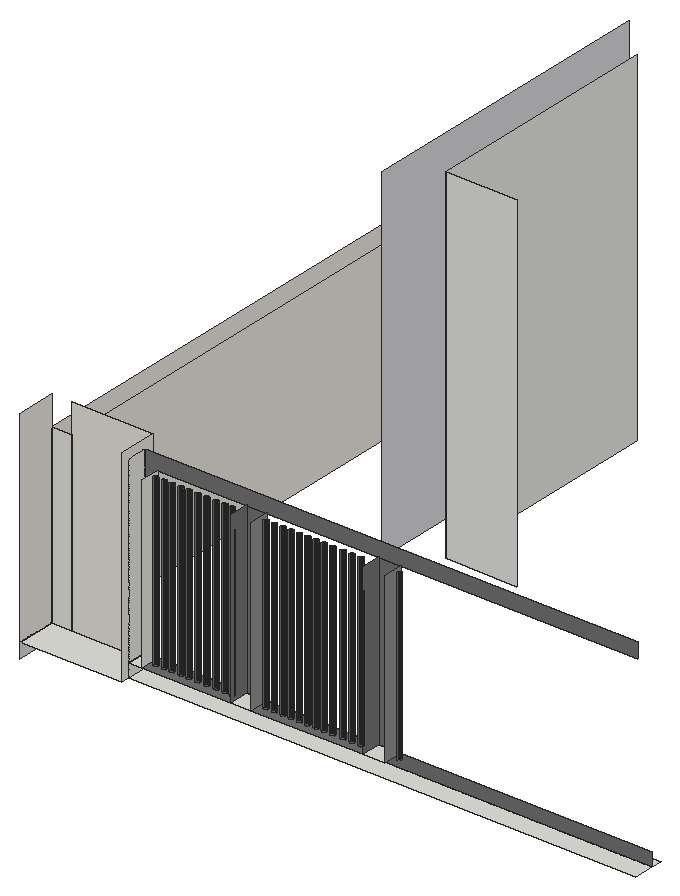
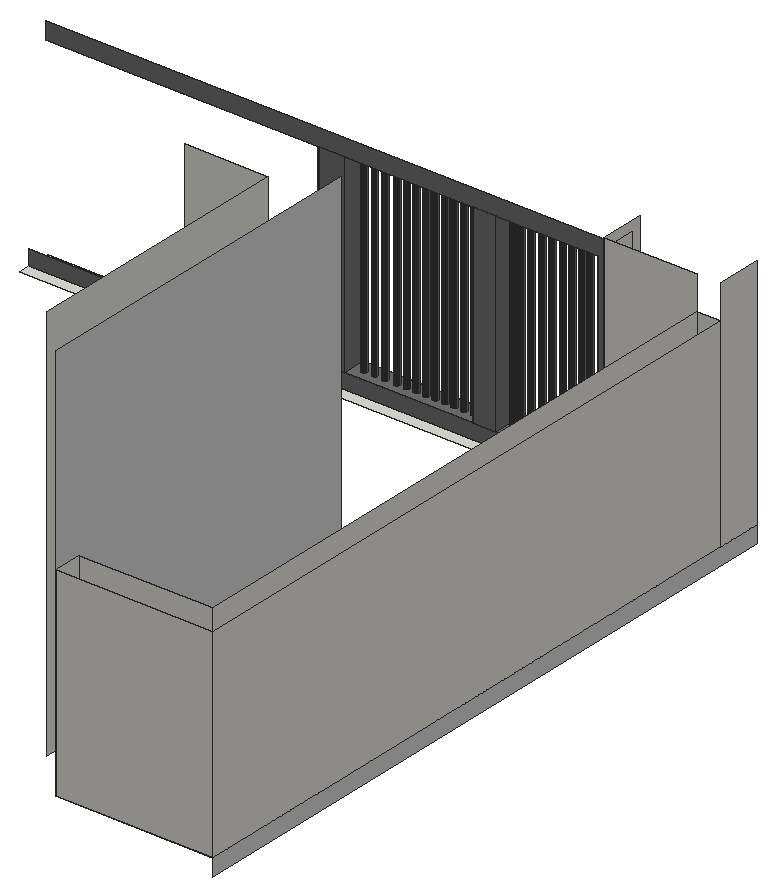
# SketchUp Ruby script. Lengths in inches.
U = 1.inch
M = Sketchup.active_model
def pt(a) = Geom::Point3d.new(a.map { |v| v * U })
def face(e, loops, mat)
  f = e.add_face(loops[0].map { |a| pt(a) })
  loops[1..].each { |l| e.add_face(l.map { |a| pt(a) }).erase! }
  f.material = f.back_material = mat if mat
  f
end
# faces: each face lists its corners as indices into pts; further lists are holes
def faces(e, pts, list, mat = nil) = list.each { |f| face(e, (f[0].is_a?(Array) ? f : [f]).map { |l| l.map { |i| pts[i] } }, mat) }
# xy, xz, yz: faces in a plane at the given z, y or x. An outline is a flat list of corners, or four numbers for a rectangle; further outlines are holes
def ring(l) = l.size == 4 ? [[l[0], l[1]], [l[2], l[1]], [l[2], l[3]], [l[0], l[3]]] : l.each_slice(2).to_a
def flat(e, list, mat, &to3) = list.each { |f| face(e, (f[0].is_a?(Array) ? f : [f]).map { |l| ring(l).map { |u, v| to3.(u, v) } }, mat) }
def xy(e, z, list, mat = nil) = flat(e, list, mat) { |x, y| [x, y, z] }
def xz(e, y, list, mat = nil) = flat(e, list, mat) { |x, z| [x, y, z] }
def yz(e, x, list, mat = nil) = flat(e, list, mat) { |y, z| [x, y, z] }
def lines(e, pts, list) = list.each { |a, b| e.add_line(pt(pts[a]), pt(pts[b])) }
# prism: a flat outline (further loops are holes) pulled along v
def prism(e, loops, v, mat = nil)
  f = face(e, loops, mat); d = Geom::Vector3d.new(v.map { |x| x * U })
  f.pushpull(f.normal.samedirection?(d) ? d.length : -d.length)
end
def box(e, o, s, mat = nil) = prism(e, [[o, [o[0] + s[0], o[1], o[2]], [o[0] + s[0], o[1] + s[1], o[2]], [o[0], o[1] + s[1], o[2]]]], [0, 0, s[2]], mat)
def at(x, y, z, deg = 0) = Geom::Transformation.translation(pt([x, y, z])) * Geom::Transformation.rotation(ORIGIN, Z_AXIS, deg.degrees)
def axes(o, x, y, z) = Geom::Transformation.new([*x, 0, *y, 0, *z, 0, *pt(o).to_a, 1])
def part(name) = M.definitions.add(name)
# library, detail: a bought-in or finely detailed component or shape, given as its bounding box
def library(name, o, s) = part(name).tap { |d| box(d.entities, o, s) }
def detail(e, o, s) = box(e.add_group.entities, o, s)
def put(e, d, t, mat = nil) = e.add_instance(d, t).tap { |i| i.material = mat if mat }
def group(e, t, mat = nil) = e.add_group.tap { |g| g.transformation = t; g.material = mat if mat }.entities
root = M.entities
M.materials.add("[Blinds Vertical Pattern]").color = [212, 212, 214]
M.materials.add("[Color M04]").color = [142, 142, 142]
M.materials.add("[Color M05]").color = [114, 114, 114]
M.materials.add("[Tile Travertine 2 inch]").color = [229, 225, 218]
xy(root,9,[[0,119.71,61.88,143.63],[61.88,125.1875,371.37,137.375],[61.88,137.375,371.37,143.63],[0,143.63,0,479.71,83.3125,479.71,83.3125,464.52,12.5625,464.52,12.5625,143.63]])
xy(root,17.125,[[61.88,125.1875,69.95,137.375],[124.17,125.1875,136.24,137.375],[204.36,125.1875,217.93,137.375]])
xy(root,17.125,[[[69.95,125.1875,124.17,137.375],[119.99,129.51,119.59,129.56,119.21,129.72,118.88,129.97,118.64,130.29,118.48,130.67,118.43,131.07,118.48,131.48,118.64,131.86,118.88,132.18,119.21,132.43,119.59,132.58,119.99,132.64,120.39,132.58,120.77,132.43,121.09,132.18,121.34,131.86,121.5,131.48,121.55,131.07,121.5,130.67,121.34,130.29,121.09,129.97,120.77,129.72,120.39,129.56],[78.3,129.51,77.9,129.56,77.52,129.72,77.2,129.97,76.95,130.29,76.79,130.67,76.74,131.07,76.79,131.48,76.95,131.86,77.2,132.18,77.52,132.43,77.9,132.58,78.3,132.64,78.71,132.58,79.08,132.43,79.41,132.18,79.66,131.86,79.8125,131.48,79.86,131.07,79.8125,130.67,79.66,130.29,79.41,129.97,79.08,129.72,78.71,129.56],[115.49,129.51,115.09,129.56,114.71,129.72,114.38,129.97,114.14,130.29,113.98,130.67,113.93,131.07,113.98,131.48,114.14,131.86,114.38,132.18,114.71,132.43,115.09,132.58,115.49,132.64,115.89,132.58,116.27,132.43,116.59,132.18,116.84,131.86,117,131.48,117.05,131.07,117,130.67,116.84,130.29,116.59,129.97,116.27,129.72,115.89,129.56],[83.3,129.51,82.9,129.56,82.52,129.72,82.2,129.97,81.95,130.29,81.79,130.67,81.74,131.07,81.79,131.48,81.95,131.86,82.2,132.18,82.52,132.43,82.9,132.58,83.3,132.64,83.71,132.58,84.08,132.43,84.41,132.18,84.66,131.86,84.8125,131.48,84.86,131.07,84.8125,130.67,84.66,130.29,84.41,129.97,84.08,129.72,83.71,129.56],[110.11,129.51,109.71,129.56,109.33,129.72,109.01,129.97,108.76,130.29,108.61,130.67,108.55,131.07,108.61,131.48,108.76,131.86,109.01,132.18,109.33,132.43,109.71,132.58,110.11,132.64,110.52,132.58,110.9,132.43,111.22,132.18,111.47,131.86,111.625,131.48,111.68,131.07,111.625,130.67,111.47,130.29,111.22,129.97,110.9,129.72,110.52,129.56],[88.61,129.51,88.21,129.56,87.83,129.72,87.51,129.97,87.26,130.29,87.11,130.67,87.05,131.07,87.11,131.48,87.26,131.86,87.51,132.18,87.83,132.43,88.21,132.58,88.61,132.64,89.02,132.58,89.4,132.43,89.72,132.18,89.97,131.86,90.125,131.48,90.18,131.07,90.125,130.67,89.97,130.29,89.72,129.97,89.4,129.72,89.02,129.56],[104.36,129.51,103.96,129.56,103.58,129.72,103.26,129.97,103.01,130.29,102.86,130.67,102.8,131.07,102.86,131.48,103.01,131.86,103.26,132.18,103.58,132.43,103.96,132.58,104.36,132.64,104.77,132.58,105.15,132.43,105.47,132.18,105.72,131.86,105.875,131.48,105.93,131.07,105.875,130.67,105.72,130.29,105.47,129.97,105.15,129.72,104.77,129.56],[93.43,129.51,93.02,129.56,92.65,129.72,92.32,129.97,92.07,130.29,91.92,130.67,91.86,131.07,91.92,131.48,92.07,131.86,92.32,132.18,92.65,132.43,93.02,132.58,93.43,132.64,93.83,132.58,94.21,132.43,94.53,132.18,94.78,131.86,94.9375,131.48,94.99,131.07,94.9375,130.67,94.78,130.29,94.53,129.97,94.21,129.72,93.83,129.56],[98.93,129.51,98.52,129.56,98.15,129.72,97.82,129.97,97.57,130.29,97.42,130.67,97.36,131.07,97.42,131.48,97.57,131.86,97.82,132.18,98.15,132.43,98.52,132.58,98.93,132.64,99.33,132.58,99.71,132.43,100.03,132.18,100.28,131.86,100.4375,131.48,100.49,131.07,100.4375,130.67,100.28,130.29,100.03,129.97,99.71,129.72,99.33,129.56],[73.24,129.51,72.84,129.56,72.46,129.72,72.13,129.97,71.89,130.29,71.73,130.67,71.68,131.07,71.73,131.48,71.89,131.86,72.13,132.18,72.46,132.43,72.84,132.58,73.24,132.64,73.64,132.58,74.02,132.43,74.34,132.18,74.59,131.86,74.75,131.48,74.8,131.07,74.75,130.67,74.59,130.29,74.34,129.97,74.02,129.72,73.64,129.56]],[[136.24,125.1875,204.36,137.375],[140.68,129.51,140.27,129.56,139.9,129.72,139.57,129.97,139.32,130.29,139.17,130.67,139.11,131.07,139.17,131.48,139.32,131.86,139.57,132.18,139.9,132.43,140.27,132.58,140.68,132.64,141.08,132.58,141.46,132.43,141.78,132.18,142.03,131.86,142.1875,131.48,142.24,131.07,142.1875,130.67,142.03,130.29,141.78,129.97,141.46,129.72,141.08,129.56],[145.74,129.51,145.34,129.56,144.96,129.72,144.63,129.97,144.39,130.29,144.23,130.67,144.18,131.07,144.23,131.48,144.39,131.86,144.63,132.18,144.96,132.43,145.34,132.58,145.74,132.64,146.14,132.58,146.52,132.43,146.84,132.18,147.09,131.86,147.25,131.48,147.3,131.07,147.25,130.67,147.09,130.29,146.84,129.97,146.52,129.72,146.14,129.56],[150.8,129.51,150.4,129.56,150.02,129.72,149.7,129.97,149.45,130.29,149.29,130.67,149.24,131.07,149.29,131.48,149.45,131.86,149.7,132.18,150.02,132.43,150.4,132.58,150.8,132.64,151.21,132.58,151.58,132.43,151.91,132.18,152.16,131.86,152.3125,131.48,152.36,131.07,152.3125,130.67,152.16,130.29,151.91,129.97,151.58,129.72,151.21,129.56],[155.86,129.51,155.46,129.56,155.08,129.72,154.76,129.97,154.51,130.29,154.36,130.67,154.3,131.07,154.36,131.48,154.51,131.86,154.76,132.18,155.08,132.43,155.46,132.58,155.86,132.64,156.27,132.58,156.65,132.43,156.97,132.18,157.22,131.86,157.375,131.48,157.43,131.07,157.375,130.67,157.22,130.29,156.97,129.97,156.65,129.72,156.27,129.56],[160.93,129.51,160.52,129.56,160.15,129.72,159.82,129.97,159.57,130.29,159.42,130.67,159.36,131.07,159.42,131.48,159.57,131.86,159.82,132.18,160.15,132.43,160.52,132.58,160.93,132.64,161.33,132.58,161.71,132.43,162.03,132.18,162.28,131.86,162.4375,131.48,162.49,131.07,162.4375,130.67,162.28,130.29,162.03,129.97,161.71,129.72,161.33,129.56],[165.99,129.51,165.59,129.56,165.21,129.72,164.88,129.97,164.64,130.29,164.48,130.67,164.43,131.07,164.48,131.48,164.64,131.86,164.88,132.18,165.21,132.43,165.59,132.58,165.99,132.64,166.39,132.58,166.77,132.43,167.09,132.18,167.34,131.86,167.5,131.48,167.55,131.07,167.5,130.67,167.34,130.29,167.09,129.97,166.77,129.72,166.39,129.56],[171.05,129.51,170.65,129.56,170.27,129.72,169.95,129.97,169.7,130.29,169.54,130.67,169.49,131.07,169.54,131.48,169.7,131.86,169.95,132.18,170.27,132.43,170.65,132.58,171.05,132.64,171.46,132.58,171.83,132.43,172.16,132.18,172.41,131.86,172.5625,131.48,172.61,131.07,172.5625,130.67,172.41,130.29,172.16,129.97,171.83,129.72,171.46,129.56],[176.11,129.51,175.71,129.56,175.33,129.72,175.01,129.97,174.76,130.29,174.61,130.67,174.55,131.07,174.61,131.48,174.76,131.86,175.01,132.18,175.33,132.43,175.71,132.58,176.11,132.64,176.52,132.58,176.9,132.43,177.22,132.18,177.47,131.86,177.625,131.48,177.68,131.07,177.625,130.67,177.47,130.29,177.22,129.97,176.9,129.72,176.52,129.56],[181.18,129.51,180.77,129.56,180.4,129.72,180.07,129.97,179.82,130.29,179.67,130.67,179.61,131.07,179.67,131.48,179.82,131.86,180.07,132.18,180.4,132.43,180.77,132.58,181.18,132.64,181.58,132.58,181.96,132.43,182.28,132.18,182.53,131.86,182.6875,131.48,182.74,131.07,182.6875,130.67,182.53,130.29,182.28,129.97,181.96,129.72,181.58,129.56],[187.68,129.51,187.27,129.56,186.9,129.72,186.57,129.97,186.32,130.29,186.17,130.67,186.11,131.07,186.17,131.48,186.32,131.86,186.57,132.18,186.9,132.43,187.27,132.58,187.68,132.64,188.08,132.58,188.46,132.43,188.78,132.18,189.03,131.86,189.1875,131.48,189.24,131.07,189.1875,130.67,189.03,130.29,188.78,129.97,188.46,129.72,188.08,129.56],[193.18,129.51,192.77,129.56,192.4,129.72,192.07,129.97,191.82,130.29,191.67,130.67,191.61,131.07,191.67,131.48,191.82,131.86,192.07,132.18,192.4,132.43,192.77,132.58,193.18,132.64,193.58,132.58,193.96,132.43,194.28,132.18,194.53,131.86,194.6875,131.48,194.74,131.07,194.6875,130.67,194.53,130.29,194.28,129.97,193.96,129.72,193.58,129.56],[198.68,129.51,198.27,129.56,197.9,129.72,197.57,129.97,197.32,130.29,197.17,130.67,197.11,131.07,197.17,131.48,197.32,131.86,197.57,132.18,197.9,132.43,198.27,132.58,198.68,132.64,199.08,132.58,199.46,132.43,199.78,132.18,200.03,131.86,200.1875,131.48,200.24,131.07,200.1875,130.67,200.03,130.29,199.78,129.97,199.46,129.72,199.08,129.56]]],"[Color M05]")
xz(root,137.375,[[61.88,9,371.37,17.125],[61.88,17.125,61.88,128.625,362.74,128.625,362.74,119.59,69.95,119.59,69.95,17.125],[124.17,17.125,136.24,119.59],[204.36,17.125,217.93,119.59]],"[Color M05]")
xz(root,143.63,[[0,9,12.5625,116.1875]])
xz(root,143.63,[[12.5625,9,61.88,133.9375]],"[Tile Travertine 2 inch]")
xz(root,309.84,[[107.23,9,151.04,220]])
xz(root,464.52,[[12.5625,9,83.3125,116.1875]],"[Tile Travertine 2 inch]")
xz(root,479.71,[[0,9,83.3125,116.1875]],"[Tile Travertine 2 inch]")
yz(root,0,[[119.71,0,479.71,9]],"[Blinds Vertical Pattern]")
yz(root,0,[[119.71,9,143.63,133.9375],[143.63,9,479.71,116.1875]],"[Tile Travertine 2 inch]")
yz(root,12.5625,[[143.63,9,464.52,116.1875]],"[Tile Travertine 2 inch]")
yz(root,61.88,[[125.1875,9,137.375,17.125],[125.1875,17.125,137.375,128.625]])
yz(root,61.88,[[119.71,9,125.1875,9,125.1875,128.625,137.375,128.625,137.375,9,143.63,9,143.63,133.9375,119.71,133.9375]],"[Tile Travertine 2 inch]")
yz(root,69.95,[[125.1875,17.125,137.375,119.59]])
yz(root,83.3125,[[464.52,9,479.71,116.1875]])
yz(root,83.3125,[[291.34,9,291.34,220,479.71,220,479.71,116.1875,464.52,116.1875,464.52,9]],"[Blinds Vertical Pattern]")
yz(root,107.23,[[309.84,9,455.8,220]])
yz(root,124.17,[[125.1875,17.125,137.375,119.59]],"[Color M05]")
yz(root,136.24,[[125.1875,17.125,137.375,119.59]],"[Color M04]")
yz(root,204.36,[[125.1875,17.125,137.375,119.59]],"[Color M05]")
yz(root,217.93,[[125.1875,17.125,137.375,119.59]],"[Color M04]")
p = [[79.86,131.07,17.125],[79.8125,131.48,17.125],[79.8125,131.48,119.59],[79.86,131.07,119.59],[81.79,131.48,17.125],[81.74,131.07,17.125],
  [81.74,131.07,119.59],[81.79,131.48,119.59],[84.86,131.07,17.125],[84.8125,131.48,17.125],[84.8125,131.48,119.59],[84.86,131.07,119.59],
  [87.11,131.48,17.125],[87.05,131.07,17.125],[87.05,131.07,119.59],[87.11,131.48,119.59],[90.18,131.07,17.125],[90.125,131.48,17.125],
  [90.125,131.48,119.59],[90.18,131.07,119.59],[91.92,131.48,17.125],[91.86,131.07,17.125],[91.86,131.07,119.59],[91.92,131.48,119.59],
  [94.99,131.07,17.125],[94.9375,131.48,17.125],[94.9375,131.48,119.59],[94.99,131.07,119.59],[97.42,131.48,17.125],[97.36,131.07,17.125],
  [97.36,131.07,119.59],[97.42,131.48,119.59],[100.49,131.07,17.125],[100.4375,131.48,17.125],[100.4375,131.48,119.59],[100.49,131.07,119.59],
  [102.86,131.48,17.125],[102.8,131.07,17.125],[102.8,131.07,119.59],[102.86,131.48,119.59],[105.93,131.07,17.125],[105.875,131.48,17.125],
  [105.875,131.48,119.59],[105.93,131.07,119.59],[108.61,131.48,17.125],[108.55,131.07,17.125],[108.55,131.07,119.59],[108.61,131.48,119.59],
  [111.68,131.07,17.125],[111.625,131.48,17.125],[111.625,131.48,119.59],[111.68,131.07,119.59],[113.98,131.48,17.125],[113.93,131.07,17.125],
  [113.93,131.07,119.59],[113.98,131.48,119.59],[117.05,131.07,17.125],[117,131.48,17.125],[117,131.48,119.59],[117.05,131.07,119.59],
  [118.48,131.48,17.125],[118.43,131.07,17.125],[118.43,131.07,119.59],[118.48,131.48,119.59],[121.55,131.07,17.125],[121.5,131.48,17.125],
  [121.5,131.48,119.59],[121.55,131.07,119.59],[139.17,131.48,17.125],[139.11,131.07,17.125],[139.11,131.07,119.59],[139.17,131.48,119.59],
  [142.24,131.07,17.125],[142.1875,131.48,17.125],[142.1875,131.48,119.59],[142.24,131.07,119.59],[144.23,131.48,17.125],[144.18,131.07,17.125],
  [144.18,131.07,119.59],[144.23,131.48,119.59],[147.3,131.07,17.125],[147.25,131.48,17.125],[147.25,131.48,119.59],[147.3,131.07,119.59],
  [149.29,131.48,17.125],[149.24,131.07,17.125],[149.24,131.07,119.59],[149.29,131.48,119.59],[152.36,131.07,17.125],[152.3125,131.48,17.125],
  [152.3125,131.48,119.59],[152.36,131.07,119.59],[154.36,131.48,17.125],[154.3,131.07,17.125],[154.3,131.07,119.59],[154.36,131.48,119.59],
  [157.43,131.07,17.125],[157.375,131.48,17.125],[157.375,131.48,119.59],[157.43,131.07,119.59],[159.42,131.48,17.125],[159.36,131.07,17.125],
  [159.36,131.07,119.59],[159.42,131.48,119.59],[162.49,131.07,17.125],[162.4375,131.48,17.125],[162.4375,131.48,119.59],[162.49,131.07,119.59],
  [164.48,131.48,17.125],[164.43,131.07,17.125],[164.43,131.07,119.59],[164.48,131.48,119.59],[167.55,131.07,17.125],[167.5,131.48,17.125],
  [167.5,131.48,119.59],[167.55,131.07,119.59],[169.54,131.48,17.125],[169.49,131.07,17.125],[169.49,131.07,119.59],[169.54,131.48,119.59],
  [172.61,131.07,17.125],[172.5625,131.48,17.125],[172.5625,131.48,119.59],[172.61,131.07,119.59],[174.61,131.48,17.125],[174.55,131.07,17.125],
  [174.55,131.07,119.59],[174.61,131.48,119.59],[177.68,131.07,17.125],[177.625,131.48,17.125],[177.625,131.48,119.59],[177.68,131.07,119.59],
  [179.67,131.48,17.125],[179.61,131.07,17.125],[179.61,131.07,119.59],[179.67,131.48,119.59],[182.74,131.07,17.125],[182.6875,131.48,17.125],
  [182.6875,131.48,119.59],[182.74,131.07,119.59],[186.17,131.48,17.125],[186.11,131.07,17.125],[186.11,131.07,119.59],[186.17,131.48,119.59],
  [189.24,131.07,17.125],[189.1875,131.48,17.125],[189.1875,131.48,119.59],[189.24,131.07,119.59],[191.67,131.48,17.125],[191.61,131.07,17.125],
  [191.61,131.07,119.59],[191.67,131.48,119.59],[194.74,131.07,17.125],[194.6875,131.48,17.125],[194.6875,131.48,119.59],[194.74,131.07,119.59],
  [197.17,131.48,17.125],[197.11,131.07,17.125],[197.11,131.07,119.59],[197.17,131.48,119.59],[200.24,131.07,17.125],[200.1875,131.48,17.125],
  [200.1875,131.48,119.59],[200.24,131.07,119.59],[220.73,131.48,17.125],[220.68,131.07,17.125],[220.68,131.07,119.59],[220.73,131.48,119.59],
  [71.89,131.86,17.125],[71.73,131.48,17.125],[71.73,131.48,119.59],[71.89,131.86,119.59],[74.75,131.48,17.125],[74.59,131.86,17.125],
  [74.59,131.86,119.59],[74.75,131.48,119.59],[76.95,131.86,17.125],[76.79,131.48,17.125],[76.79,131.48,119.59],[76.95,131.86,119.59],
  [79.66,131.86,17.125],[79.66,131.86,119.59],[81.95,131.86,17.125],[81.95,131.86,119.59],[84.66,131.86,17.125],[84.66,131.86,119.59],
  [87.26,131.86,17.125],[87.26,131.86,119.59],[89.97,131.86,17.125],[89.97,131.86,119.59],[92.07,131.86,17.125],[92.07,131.86,119.59],
  [94.78,131.86,17.125],[94.78,131.86,119.59],[97.57,131.86,17.125],[97.57,131.86,119.59],[100.28,131.86,17.125],[100.28,131.86,119.59],
  [103.01,131.86,17.125],[103.01,131.86,119.59],[105.72,131.86,17.125],[105.72,131.86,119.59],[108.76,131.86,17.125],[108.76,131.86,119.59],
  [111.47,131.86,17.125],[111.47,131.86,119.59],[114.14,131.86,17.125],[114.14,131.86,119.59],[116.84,131.86,17.125],[116.84,131.86,119.59],
  [118.64,131.86,17.125],[118.64,131.86,119.59],[121.34,131.86,17.125],[121.34,131.86,119.59],[139.32,131.86,17.125],[139.32,131.86,119.59],
  [142.03,131.86,17.125],[142.03,131.86,119.59],[144.39,131.86,17.125],[144.39,131.86,119.59],[147.09,131.86,17.125],[147.09,131.86,119.59],
  [149.45,131.86,17.125],[149.45,131.86,119.59],[152.16,131.86,17.125],[152.16,131.86,119.59],[154.51,131.86,17.125],[154.51,131.86,119.59],
  [157.22,131.86,17.125],[157.22,131.86,119.59],[159.57,131.86,17.125],[159.57,131.86,119.59],[162.28,131.86,17.125],[162.28,131.86,119.59],
  [164.64,131.86,17.125],[164.64,131.86,119.59],[167.34,131.86,17.125],[167.34,131.86,119.59],[169.7,131.86,17.125],[169.7,131.86,119.59],
  [172.41,131.86,17.125],[172.41,131.86,119.59],[174.76,131.86,17.125],[174.76,131.86,119.59],[177.47,131.86,17.125],[177.47,131.86,119.59],
  [179.82,131.86,17.125],[179.82,131.86,119.59],[182.53,131.86,17.125],[182.53,131.86,119.59],[186.32,131.86,17.125],[186.32,131.86,119.59],
  [189.03,131.86,17.125],[189.03,131.86,119.59],[191.82,131.86,17.125],[191.82,131.86,119.59],[194.53,131.86,17.125],[194.53,131.86,119.59],
  [197.32,131.86,17.125],[197.32,131.86,119.59],[200.03,131.86,17.125],[200.03,131.86,119.59],[220.89,131.86,17.125],[220.89,131.86,119.59],
  [72.13,132.18,17.125],[72.13,132.18,119.59],[74.34,132.18,17.125],[74.34,132.18,119.59],[77.2,132.18,17.125],[77.2,132.18,119.59],
  [79.41,132.18,17.125],[79.41,132.18,119.59],[82.2,132.18,17.125],[82.2,132.18,119.59],[84.41,132.18,17.125],[84.41,132.18,119.59],
  [87.51,132.18,17.125],[87.51,132.18,119.59],[89.72,132.18,17.125],[89.72,132.18,119.59],[92.32,132.18,17.125],[92.32,132.18,119.59],
  [94.53,132.18,17.125],[94.53,132.18,119.59],[97.82,132.18,17.125],[97.82,132.18,119.59],[100.03,132.18,17.125],[100.03,132.18,119.59],
  [103.26,132.18,17.125],[103.26,132.18,119.59],[105.47,132.18,17.125],[105.47,132.18,119.59],[109.01,132.18,17.125],[109.01,132.18,119.59],
  [111.22,132.18,17.125],[111.22,132.18,119.59],[114.38,132.18,17.125],[114.38,132.18,119.59],[116.59,132.18,17.125],[116.59,132.18,119.59],
  [118.88,132.18,17.125],[118.88,132.18,119.59],[121.09,132.18,17.125],[121.09,132.18,119.59],[139.57,132.18,17.125],[139.57,132.18,119.59],
  [141.78,132.18,17.125],[141.78,132.18,119.59],[144.63,132.18,17.125],[144.63,132.18,119.59],[146.84,132.18,17.125],[146.84,132.18,119.59],
  [149.7,132.18,17.125],[149.7,132.18,119.59],[151.91,132.18,17.125],[151.91,132.18,119.59],[154.76,132.18,17.125],[154.76,132.18,119.59],
  [156.97,132.18,17.125],[156.97,132.18,119.59],[159.82,132.18,17.125],[159.82,132.18,119.59],[162.03,132.18,17.125],[162.03,132.18,119.59],
  [164.88,132.18,17.125],[164.88,132.18,119.59],[167.09,132.18,17.125],[167.09,132.18,119.59],[169.95,132.18,17.125],[169.95,132.18,119.59],
  [172.16,132.18,17.125],[172.16,132.18,119.59],[175.01,132.18,17.125],[175.01,132.18,119.59],[177.22,132.18,17.125],[177.22,132.18,119.59],
  [180.07,132.18,17.125],[180.07,132.18,119.59],[182.28,132.18,17.125],[182.28,132.18,119.59],[186.57,132.18,17.125],[186.57,132.18,119.59],
  [188.78,132.18,17.125],[188.78,132.18,119.59],[192.07,132.18,17.125],[192.07,132.18,119.59],[194.28,132.18,17.125],[194.28,132.18,119.59],
  [197.57,132.18,17.125],[197.57,132.18,119.59],[199.78,132.18,17.125],[199.78,132.18,119.59],[221.13,132.18,17.125],[221.13,132.18,119.59],
  [72.46,132.43,17.125],[72.46,132.43,119.59],[74.02,132.43,17.125],[74.02,132.43,119.59],[77.52,132.43,17.125],[77.52,132.43,119.59],
  [79.08,132.43,17.125],[79.08,132.43,119.59],[82.52,132.43,17.125],[82.52,132.43,119.59],[84.08,132.43,17.125],[84.08,132.43,119.59],
  [87.83,132.43,17.125],[87.83,132.43,119.59],[89.4,132.43,17.125],[89.4,132.43,119.59],[92.65,132.43,17.125],[92.65,132.43,119.59],
  [94.21,132.43,17.125],[94.21,132.43,119.59],[98.15,132.43,17.125],[98.15,132.43,119.59],[99.71,132.43,17.125],[99.71,132.43,119.59],
  [103.58,132.43,17.125],[103.58,132.43,119.59],[105.15,132.43,17.125],[105.15,132.43,119.59],[109.33,132.43,17.125],[109.33,132.43,119.59],
  [110.9,132.43,17.125],[110.9,132.43,119.59],[114.71,132.43,17.125],[114.71,132.43,119.59],[116.27,132.43,17.125],[116.27,132.43,119.59],
  [119.21,132.43,17.125],[119.21,132.43,119.59],[120.77,132.43,17.125],[120.77,132.43,119.59],[139.9,132.43,17.125],[139.9,132.43,119.59],
  [141.46,132.43,17.125],[141.46,132.43,119.59],[144.96,132.43,17.125],[144.96,132.43,119.59],[146.52,132.43,17.125],[146.52,132.43,119.59],
  [150.02,132.43,17.125],[150.02,132.43,119.59],[151.58,132.43,17.125],[151.58,132.43,119.59],[155.08,132.43,17.125],[155.08,132.43,119.59],
  [156.65,132.43,17.125],[156.65,132.43,119.59],[160.15,132.43,17.125],[160.15,132.43,119.59],[161.71,132.43,17.125],[161.71,132.43,119.59],
  [165.21,132.43,17.125],[165.21,132.43,119.59],[166.77,132.43,17.125],[166.77,132.43,119.59],[170.27,132.43,17.125],[170.27,132.43,119.59],
  [171.83,132.43,17.125],[171.83,132.43,119.59],[175.33,132.43,17.125],[175.33,132.43,119.59],[176.9,132.43,17.125],[176.9,132.43,119.59],
  [180.4,132.43,17.125],[180.4,132.43,119.59],[181.96,132.43,17.125],[181.96,132.43,119.59],[186.9,132.43,17.125],[186.9,132.43,119.59],
  [188.46,132.43,17.125],[188.46,132.43,119.59],[192.4,132.43,17.125],[192.4,132.43,119.59],[193.96,132.43,17.125],[193.96,132.43,119.59],
  [197.9,132.43,17.125],[197.9,132.43,119.59],[199.46,132.43,17.125],[199.46,132.43,119.59],[221.46,132.43,17.125],[221.46,132.43,119.59],
  [72.84,132.58,17.125],[72.84,132.58,119.59],[73.64,132.58,17.125],[73.64,132.58,119.59],[77.9,132.58,17.125],[77.9,132.58,119.59],
  [78.71,132.58,17.125],[78.71,132.58,119.59],[82.9,132.58,17.125],[82.9,132.58,119.59],[83.71,132.58,17.125],[83.71,132.58,119.59],
  [88.21,132.58,17.125],[88.21,132.58,119.59],[89.02,132.58,17.125],[89.02,132.58,119.59],[93.02,132.58,17.125],[93.02,132.58,119.59],
  [93.83,132.58,17.125],[93.83,132.58,119.59],[98.52,132.58,17.125],[98.52,132.58,119.59],[99.33,132.58,17.125],[99.33,132.58,119.59],
  [103.96,132.58,17.125],[103.96,132.58,119.59],[104.77,132.58,17.125],[104.77,132.58,119.59],[109.71,132.58,17.125],[109.71,132.58,119.59],
  [110.52,132.58,17.125],[110.52,132.58,119.59],[115.09,132.58,17.125],[115.09,132.58,119.59],[115.89,132.58,17.125],[115.89,132.58,119.59],
  [119.59,132.58,17.125],[119.59,132.58,119.59],[120.39,132.58,17.125],[120.39,132.58,119.59],[140.27,132.58,17.125],[140.27,132.58,119.59],
  [141.08,132.58,17.125],[141.08,132.58,119.59],[145.34,132.58,17.125],[145.34,132.58,119.59],[146.14,132.58,17.125],[146.14,132.58,119.59],
  [150.4,132.58,17.125],[150.4,132.58,119.59],[151.21,132.58,17.125],[151.21,132.58,119.59],[155.46,132.58,17.125],[155.46,132.58,119.59],
  [156.27,132.58,17.125],[156.27,132.58,119.59],[160.52,132.58,17.125],[160.52,132.58,119.59],[161.33,132.58,17.125],[161.33,132.58,119.59],
  [165.59,132.58,17.125],[165.59,132.58,119.59],[166.39,132.58,17.125],[166.39,132.58,119.59],[170.65,132.58,17.125],[170.65,132.58,119.59],
  [171.46,132.58,17.125],[171.46,132.58,119.59],[175.71,132.58,17.125],[175.71,132.58,119.59],[176.52,132.58,17.125],[176.52,132.58,119.59],
  [180.77,132.58,17.125],[180.77,132.58,119.59],[181.58,132.58,17.125],[181.58,132.58,119.59],[187.27,132.58,17.125],[187.27,132.58,119.59],
  [188.08,132.58,17.125],[188.08,132.58,119.59],[192.77,132.58,17.125],[192.77,132.58,119.59],[193.58,132.58,17.125],[193.58,132.58,119.59],
  [198.27,132.58,17.125],[198.27,132.58,119.59],[199.08,132.58,17.125],[199.08,132.58,119.59],[221.84,132.58,17.125],[221.84,132.58,119.59],
  [73.24,132.64,17.125],[73.24,132.64,119.59],[78.3,132.64,17.125],[78.3,132.64,119.59],[83.3,132.64,17.125],[83.3,132.64,119.59],
  [88.61,132.64,17.125],[88.61,132.64,119.59],[93.43,132.64,17.125],[93.43,132.64,119.59],[98.93,132.64,17.125],[98.93,132.64,119.59],
  [104.36,132.64,17.125],[104.36,132.64,119.59],[110.11,132.64,17.125],[110.11,132.64,119.59],[115.49,132.64,17.125],[115.49,132.64,119.59],
  [119.99,132.64,17.125],[119.99,132.64,119.59],[140.68,132.64,17.125],[140.68,132.64,119.59],[145.74,132.64,17.125],[145.74,132.64,119.59],
  [150.8,132.64,17.125],[150.8,132.64,119.59],[155.86,132.64,17.125],[155.86,132.64,119.59],[160.93,132.64,17.125],[160.93,132.64,119.59],
  [165.99,132.64,17.125],[165.99,132.64,119.59],[171.05,132.64,17.125],[171.05,132.64,119.59],[176.11,132.64,17.125],[176.11,132.64,119.59],
  [181.18,132.64,17.125],[181.18,132.64,119.59],[187.68,132.64,17.125],[187.68,132.64,119.59],[193.18,132.64,17.125],[193.18,132.64,119.59],
  [198.68,132.64,17.125],[198.68,132.64,119.59],[222.24,132.64,17.125],[222.24,132.64,119.59]]
faces(root,p,[[0,1,2,3],[4,5,6,7],[8,9,10,11],[12,13,14,15],[16,17,18,19],[20,21,22,23],[24,25,26,27],[28,29,30,31],
  [32,33,34,35],[36,37,38,39],[40,41,42,43],[44,45,46,47],[48,49,50,51],[52,53,54,55],[56,57,58,59],[60,61,62,63],
  [64,65,66,67],[68,69,70,71],[72,73,74,75],[76,77,78,79],[80,81,82,83],[84,85,86,87],[88,89,90,91],[92,93,94,95],
  [96,97,98,99],[100,101,102,103],[104,105,106,107],[108,109,110,111],[112,113,114,115],[116,117,118,119],[120,121,122,123],[124,125,126,127],
  [128,129,130,131],[132,133,134,135],[136,137,138,139],[140,141,142,143],[144,145,146,147],[148,149,150,151],[152,153,154,155],[156,157,158,159],
  [160,161,162,163],[164,165,166,167],[168,169,170,171],[172,173,174,175],[176,177,178,179],[1,180,181,2],[182,4,7,183],[9,184,185,10],
  [186,12,15,187],[17,188,189,18],[190,20,23,191],[25,192,193,26],[194,28,31,195],[33,196,197,34],[198,36,39,199],[41,200,201,42],
  [202,44,47,203],[49,204,205,50],[206,52,55,207],[57,208,209,58],[210,60,63,211],[65,212,213,66],[214,68,71,215],[73,216,217,74],
  [218,76,79,219],[81,220,221,82],[222,84,87,223],[89,224,225,90],[226,92,95,227],[97,228,229,98],[230,100,103,231],[105,232,233,106],
  [234,108,111,235],[113,236,237,114],[238,116,119,239],[121,240,241,122],[242,124,127,243],[129,244,245,130],[246,132,135,247],[137,248,249,138],
  [250,140,143,251],[145,252,253,146],[254,148,151,255],[153,256,257,154],[258,156,159,259],[161,260,261,162],[262,164,167,263],[264,168,171,265],
  [173,266,267,174],[268,176,179,269],[180,270,271,181],[272,182,183,273],[184,274,275,185],[276,186,187,277],[188,278,279,189],[280,190,191,281],
  [192,282,283,193],[284,194,195,285],[196,286,287,197],[288,198,199,289],[200,290,291,201],[292,202,203,293],[204,294,295,205],[296,206,207,297],
  [208,298,299,209],[300,210,211,301],[212,302,303,213],[304,214,215,305],[216,306,307,217],[308,218,219,309],[220,310,311,221],[312,222,223,313],
  [224,314,315,225],[316,226,227,317],[228,318,319,229],[320,230,231,321],[232,322,323,233],[324,234,235,325],[236,326,327,237],[328,238,239,329],
  [240,330,331,241],[332,242,243,333],[244,334,335,245],[336,246,247,337],[248,338,339,249],[340,250,251,341],[252,342,343,253],[344,254,255,345],
  [256,346,347,257],[348,258,259,349],[260,350,351,261],[352,262,263,353],[354,264,265,355],[266,356,357,267],[358,268,269,359],[270,360,361,271],
  [362,272,273,363],[274,364,365,275],[366,276,277,367],[278,368,369,279],[370,280,281,371],[282,372,373,283],[374,284,285,375],[286,376,377,287],
  [378,288,289,379],[290,380,381,291],[382,292,293,383],[294,384,385,295],[386,296,297,387],[298,388,389,299],[390,300,301,391],[302,392,393,303],
  [394,304,305,395],[306,396,397,307],[398,308,309,399],[310,400,401,311],[402,312,313,403],[314,404,405,315],[406,316,317,407],[318,408,409,319],
  [410,320,321,411],[322,412,413,323],[414,324,325,415],[326,416,417,327],[418,328,329,419],[330,420,421,331],[422,332,333,423],[334,424,425,335],
  [426,336,337,427],[338,428,429,339],[430,340,341,431],[342,432,433,343],[434,344,345,435],[346,436,437,347],[438,348,349,439],[350,440,441,351],
  [442,352,353,443],[444,354,355,445],[356,446,447,357],[448,358,359,449],[360,450,451,361],[452,362,363,453],[364,454,455,365],[456,366,367,457],
  [368,458,459,369],[460,370,371,461],[372,462,463,373],[464,374,375,465],[376,466,467,377],[468,378,379,469],[380,470,471,381],[472,382,383,473],
  [384,474,475,385],[476,386,387,477],[388,478,479,389],[480,390,391,481],[392,482,483,393],[484,394,395,485],[396,486,487,397],[488,398,399,489],
  [400,490,491,401],[492,402,403,493],[404,494,495,405],[496,406,407,497],[408,498,499,409],[500,410,411,501],[412,502,503,413],[504,414,415,505],
  [416,506,507,417],[508,418,419,509],[420,510,511,421],[512,422,423,513],[424,514,515,425],[516,426,427,517],[428,518,519,429],[520,430,431,521],
  [432,522,523,433],[524,434,435,525],[436,526,527,437],[528,438,439,529],[440,530,531,441],[532,442,443,533],[534,444,445,535],[446,534,535,447],
  [536,448,449,537],[450,536,537,451],[538,452,453,539],[454,538,539,455],[540,456,457,541],[458,540,541,459],[542,460,461,543],[462,542,543,463],
  [544,464,465,545],[466,544,545,467],[546,468,469,547],[470,546,547,471],[548,472,473,549],[474,548,549,475],[550,476,477,551],[478,550,551,479],
  [552,480,481,553],[482,552,553,483],[554,484,485,555],[486,554,555,487],[556,488,489,557],[490,556,557,491],[558,492,493,559],[494,558,559,495],
  [560,496,497,561],[498,560,561,499],[562,500,501,563],[502,562,563,503],[564,504,505,565],[506,564,565,507],[566,508,509,567],[510,566,567,511],
  [568,512,513,569],[514,568,569,515],[570,516,517,571],[518,570,571,519],[572,520,521,573],[522,572,573,523],[574,524,525,575],[526,574,575,527],
  [576,528,529,577],[530,576,577,531],[578,532,533,579]],"[Color M05]")
